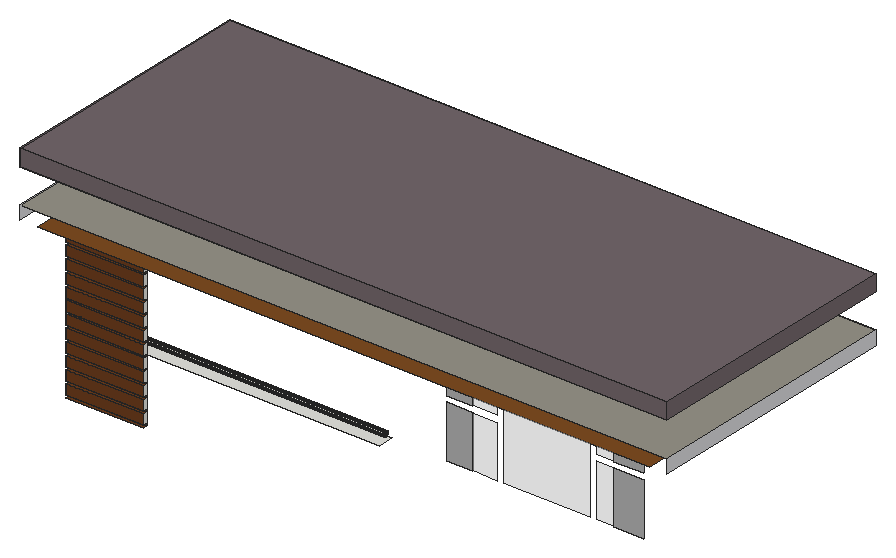
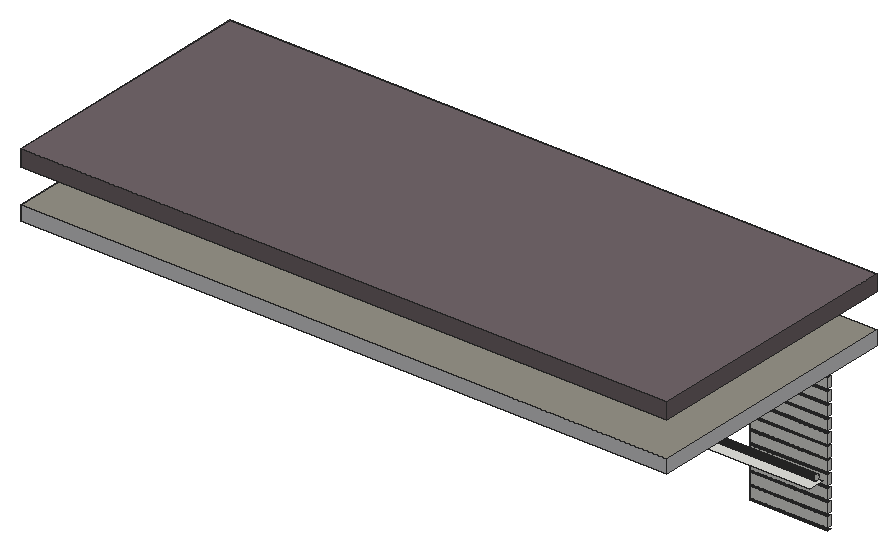
# SketchUp Ruby script. Lengths in inches.
U = 1.inch
M = Sketchup.active_model
def pt(a) = Geom::Point3d.new(a.map { |v| v * U })
def face(e, loops, mat)
  f = e.add_face(loops[0].map { |a| pt(a) })
  loops[1..].each { |l| e.add_face(l.map { |a| pt(a) }).erase! }
  f.material = f.back_material = mat if mat
  f
end
# faces: each face lists its corners as indices into pts; further lists are holes
def faces(e, pts, list, mat = nil) = list.each { |f| face(e, (f[0].is_a?(Array) ? f : [f]).map { |l| l.map { |i| pts[i] } }, mat) }
# xy, xz, yz: faces in a plane at the given z, y or x. An outline is a flat list of corners, or four numbers for a rectangle; further outlines are holes
def ring(l) = l.size == 4 ? [[l[0], l[1]], [l[2], l[1]], [l[2], l[3]], [l[0], l[3]]] : l.each_slice(2).to_a
def flat(e, list, mat, &to3) = list.each { |f| face(e, (f[0].is_a?(Array) ? f : [f]).map { |l| ring(l).map { |u, v| to3.(u, v) } }, mat) }
def xy(e, z, list, mat = nil) = flat(e, list, mat) { |x, y| [x, y, z] }
def xz(e, y, list, mat = nil) = flat(e, list, mat) { |x, z| [x, y, z] }
def yz(e, x, list, mat = nil) = flat(e, list, mat) { |y, z| [x, y, z] }
def lines(e, pts, list) = list.each { |a, b| e.add_line(pt(pts[a]), pt(pts[b])) }
# prism: a flat outline (further loops are holes) pulled along v
def prism(e, loops, v, mat = nil)
  f = face(e, loops, mat); d = Geom::Vector3d.new(v.map { |x| x * U })
  f.pushpull(f.normal.samedirection?(d) ? d.length : -d.length)
end
def box(e, o, s, mat = nil) = prism(e, [[o, [o[0] + s[0], o[1], o[2]], [o[0] + s[0], o[1] + s[1], o[2]], [o[0], o[1] + s[1], o[2]]]], [0, 0, s[2]], mat)
def at(x, y, z, deg = 0) = Geom::Transformation.translation(pt([x, y, z])) * Geom::Transformation.rotation(ORIGIN, Z_AXIS, deg.degrees)
def axes(o, x, y, z) = Geom::Transformation.new([*x, 0, *y, 0, *z, 0, *pt(o).to_a, 1])
def part(name) = M.definitions.add(name)
# library, detail: a bought-in or finely detailed component or shape, given as its bounding box
def library(name, o, s) = part(name).tap { |d| box(d.entities, o, s) }
def detail(e, o, s) = box(e.add_group.entities, o, s)
def put(e, d, t, mat = nil) = e.add_instance(d, t).tap { |i| i.material = mat if mat }
def group(e, t, mat = nil) = e.add_group.tap { |g| g.transformation = t; g.material = mat if mat }.entities
root = M.entities
M.materials.add("[Asphalt New]").color = [114, 102, 106]
M.materials.add("[Blinds Vertical Pattern]").color = [212, 212, 214]
M.materials.add("[Blinds Vertical Stripe Gray]1").color = [175, 175, 175]
M.materials.add("[Color M07]").color = [58, 58, 58]
M.materials.add("[Formica Graystone]3").color = [149, 146, 135]
M.materials.add("[Formica Laminate Dark]").color = [50, 53, 60]
M.materials.add("[Quartz Light Brown]").color = [224, 207, 171]
M.materials.add("[Terrazzo Tile Light]").color = [219, 217, 210]
M.materials.add("[Translucent Glass Gray]1").color = [224, 224, 224]
M.materials["[Translucent Glass Gray]1"].alpha = 0.5
M.materials.add("[Wood Cherry Original]").color = [107, 60, 29]
M.materials.add("[Wood Floor Parquet]").color = [124, 76, 33]
xy(root,275.9375,[[110.71,220.49,195.83,224.74]],"[Wood Cherry Original]")
xy(root,278.71,[[110.71,220.49,195.02,224.74],[195.02,220.49,195.83,224.74]],"[Wood Cherry Original]")
xy(root,289.6875,[[110.71,220.49,195.83,224.74]],"[Wood Cherry Original]")
xy(root,292.46,[[110.71,220.49,195.02,224.74],[195.02,220.49,195.83,224.74]],"[Wood Cherry Original]")
xy(root,303.4375,[[110.71,220.49,195.83,224.74]],"[Wood Cherry Original]")
xy(root,306.21,[[110.71,220.49,195.02,224.74],[195.02,220.49,195.83,224.74]],"[Wood Cherry Original]")
xy(root,317.1875,[[110.71,220.49,195.83,224.74]],"[Wood Cherry Original]")
xy(root,319.83,[[110.71,220.49,195.02,224.74],[195.02,220.49,195.83,224.74]],"[Wood Cherry Original]")
xy(root,330.8125,[[110.71,220.49,195.83,224.74]],"[Wood Cherry Original]")
xy(root,333.46,[[110.71,220.49,195.02,224.74],[195.02,220.49,195.83,224.74]],"[Wood Cherry Original]")
xy(root,334.75,[[102.3,241.34,438.59,258.82]])
xy(root,344.4375,[[110.71,220.49,195.83,224.74]],"[Wood Cherry Original]")
xy(root,347.08,[[110.71,220.49,195.02,224.74],[195.02,220.49,195.83,224.74]],"[Wood Cherry Original]")
xy(root,358.0625,[[110.71,220.49,195.83,224.74]],"[Wood Cherry Original]")
xy(root,360.71,[[110.71,220.49,195.02,224.74],[195.02,220.49,195.83,224.74]],"[Wood Cherry Original]")
xy(root,371.6875,[[110.71,220.49,195.83,224.74]],"[Wood Cherry Original]")
xy(root,374.33,[[110.71,220.49,195.02,224.74],[195.02,220.49,195.83,224.74]],"[Wood Cherry Original]")
xy(root,385.3125,[[110.71,220.49,195.83,224.74]],"[Wood Cherry Original]")
xy(root,387.96,[[110.71,220.49,195.02,224.74],[195.02,220.49,195.83,224.74]],"[Wood Cherry Original]")
xy(root,398.9375,[[110.71,220.49,195.83,224.74]],"[Wood Cherry Original]")
xy(root,401.58,[[110.71,220.49,195.02,224.74],[195.02,220.49,195.83,224.74]],"[Wood Cherry Original]")
xy(root,412.5625,[[110.71,220.49,195.83,224.74]],"[Wood Cherry Original]")
xy(root,415.21,[[110.71,220.49,195.02,224.74],[195.02,220.49,195.83,224.74]],"[Wood Cherry Original]")
xy(root,426.1875,[[110.71,220.49,195.83,224.74]],"[Wood Cherry Original]")
xy(root,428.83,[[110.71,220.49,195.02,224.74],[195.02,220.49,195.83,224.74]],"[Wood Cherry Original]")
xy(root,430,[[488.69,241.34,724.51,258.97]],"[Quartz Light Brown]")
xy(root,439.8125,[[110.71,220.49,195.83,224.74]],"[Wood Cherry Original]")
xy(root,442.46,[[110.71,220.49,195.02,224.74],[195.02,220.49,195.83,224.74]],"[Wood Cherry Original]")
xy(root,453.4375,[[83.3125,217.06,102.3,233.68],[102.3,217.06,102.3,233.68,204.43,233.68,204.43,217.06,195.83,217.06,195.83,224.74,110.71,224.74,110.71,217.06],[110.71,220.49,195.83,224.74],[110.71,220.49,195.83,224.74],[83.3125,233.68,102.3,241.34],
  [83.3125,241.34,102.3,355.28],[438.59,241.34,774.88,305.05],[774.88,241.34,793.87,305.05],[438.59,305.05,455.13,355.28],[455.13,305.05,774.88,355.28],
  [774.88,305.05,793.87,355.28],[83.3125,355.28,102.3,479.71],[102.3,355.28,438.59,460.72],[438.59,355.28,455.13,460.72],[455.13,355.28,774.88,460.72],
  [774.88,355.28,793.87,479.71],[102.3,460.72,438.59,479.71],[438.59,460.72,455.13,479.71],[455.13,460.72,774.88,479.71]])
xy(root,453.4375,[[102.3,191.84,102.3,217.06,110.71,217.06,110.71,220.49,195.83,220.49,195.83,217.06,204.43,217.06,204.43,233.68,102.3,233.68,102.3,355.28,438.59,355.28,438.59,241.34,774.88,241.34,774.88,191.84]],"[Wood Floor Parquet]")
xy(root,468.5,[[164.19,296.67,679.38,375.05]])
xy(root,468.5,[[[83.3125,191.84,793.87,479.71],[164.19,296.67,679.38,375.05]]],"[Formica Graystone]3")
xy(root,506.5,[[164.19,296.67,679.38,375.05]])
xy(root,506.5,[[83.3125,191.84,83.3125,479.71,164.19,479.71,164.19,296.67,679.38,296.67,679.38,479.71,793.87,479.71,793.87,191.84],[164.19,375.05,679.38,479.71]],"[Asphalt New]")
xy(root,524.25,[[83.3125,191.84,793.87,479.71]],"[Asphalt New]")
xz(root,191.84,[[83.3125,506.5,793.87,524.25]],"[Asphalt New]")
xz(root,220.49,[[110.71,278.71,195.83,289.6875],[110.71,292.46,195.83,303.4375],[110.71,306.21,195.83,317.1875],[110.71,319.83,195.83,330.8125],[110.71,333.46,195.83,344.4375],
  [110.71,347.08,195.83,358.0625],[110.71,360.71,195.83,371.6875],[110.71,374.33,195.83,385.3125],[110.71,387.96,195.83,398.9375],[110.71,401.58,195.83,412.5625],
  [110.71,415.21,195.83,426.1875],[110.71,428.83,195.83,439.8125],[110.71,442.46,195.83,453.4375]],"[Wood Cherry Original]")
xz(root,224.74,[[110.71,278.71,195.83,289.6875],[110.71,292.46,195.83,303.4375],[110.71,306.21,195.83,317.1875],[110.71,319.83,195.83,330.8125],[110.71,333.46,195.83,344.4375],
  [110.71,347.08,195.83,358.0625],[110.71,360.71,195.83,371.6875],[110.71,374.33,195.83,385.3125],[110.71,387.96,195.83,398.9375],[110.71,401.58,195.83,412.5625],
  [110.71,415.21,195.83,426.1875],[110.71,428.83,195.83,439.8125],[110.71,442.46,195.83,453.4375]])
xz(root,224.74,[[110.71,275.9375,195.83,278.71],[110.71,289.6875,195.83,292.46],[110.71,303.4375,195.83,306.21],[110.71,317.1875,195.83,319.83],[110.71,330.8125,195.83,333.46],
  [110.71,344.4375,195.83,347.08],[110.71,358.0625,195.83,360.71],[110.71,371.6875,195.83,374.33],[110.71,385.3125,195.83,387.96],[110.71,398.9375,195.83,401.58],
  [110.71,412.5625,195.83,415.21],[110.71,426.1875,195.83,428.83],[110.71,439.8125,195.83,442.46]],"[Color M07]")
xz(root,258.97,[[497.89,332.38,526.43,390.39],[682.12,332.38,715.3125,390.39],[497.89,396.84,526.43,420.81],[682.12,396.84,715.3125,420.81]],"[Blinds Vertical Stripe Gray]1")
xz(root,258.97,[[526.43,332.38,554.98,390.39],[561.48,332.38,656.23,420.81],[662.73,332.38,682.12,390.39],[526.43,396.84,554.98,420.81],[662.73,396.84,682.12,420.81]],"[Translucent Glass Gray]1")
xz(root,296.67,[[164.19,468.5,679.38,506.5]],"[Formica Laminate Dark]")
xz(root,375.05,[[164.19,468.5,679.38,506.5]],"[Formica Laminate Dark]")
xz(root,479.71,[[83.3125,506.5,793.87,524.25]],"[Asphalt New]")
xz(root,479.71,[[83.3125,453.4375,793.87,468.5]],"[Blinds Vertical Pattern]")
yz(root,83.3125,[[191.84,506.5,479.71,524.25]],"[Asphalt New]")
yz(root,83.3125,[[191.84,453.4375,479.71,468.5]],"[Blinds Vertical Pattern]")
yz(root,102.3,[[250.08,339.44,249.34,339.54,248.64,339.83,248.05,340.28,247.59,340.88,247.3,341.57,247.21,342.32,247.3,343.06,247.59,343.75,248.05,344.35,248.64,344.81,249.34,345.09,250.08,345.19,250.83,345.09,251.52,344.81,252.11,344.35,252.57,343.75,252.86,343.06,252.96,342.32,252.86,341.57,252.57,340.88,252.11,340.28,251.52,339.83,250.83,339.54]])
yz(root,110.71,[[220.49,278.71,224.74,289.6875],[220.49,292.46,224.74,303.4375],[220.49,306.21,224.74,317.1875],[220.49,319.83,224.74,330.8125],[220.49,333.46,224.74,344.4375],
  [220.49,347.08,224.74,358.0625],[220.49,360.71,224.74,371.6875],[220.49,374.33,224.74,385.3125],[220.49,387.96,224.74,398.9375],[220.49,401.58,224.74,412.5625],
  [220.49,415.21,224.74,426.1875],[220.49,428.83,224.74,439.8125],[220.49,442.46,224.74,453.4375]])
yz(root,164.19,[[296.67,468.5,375.05,506.5]],"[Formica Laminate Dark]")
yz(root,195.83,[[220.49,278.71,224.74,289.6875],[220.49,292.46,224.74,303.4375],[220.49,306.21,224.74,317.1875],[220.49,319.83,224.74,330.8125],[220.49,333.46,224.74,344.4375],
  [220.49,347.08,224.74,358.0625],[220.49,360.71,224.74,371.6875],[220.49,374.33,224.74,385.3125],[220.49,387.96,224.74,398.9375],[220.49,401.58,224.74,412.5625],
  [220.49,415.21,224.74,426.1875],[220.49,428.83,224.74,439.8125],[220.49,442.46,224.74,453.4375]])
yz(root,679.38,[[296.67,468.5,375.05,506.5]],"[Formica Laminate Dark]")
yz(root,793.87,[[191.84,506.5,479.71,524.25]],"[Asphalt New]")
yz(root,793.87,[[191.84,453.4375,479.71,468.5]],"[Blinds Vertical Pattern]")
p = [[102.3,249.34,339.54],[102.3,250.08,339.44],[438.59,250.08,339.44],[438.59,249.34,339.54],[102.3,250.83,339.54],[438.59,250.83,339.54],
  [102.3,248.64,339.83],[438.59,248.64,339.83],[102.3,251.52,339.83],[438.59,251.52,339.83],[102.3,248.05,340.28],[438.59,248.05,340.28],
  [102.3,252.11,340.28],[438.59,252.11,340.28],[102.3,247.59,340.88],[438.59,247.59,340.88],[102.3,252.57,340.88],[438.59,252.57,340.88],
  [102.3,247.3,341.57],[438.59,247.3,341.57],[102.3,252.86,341.57],[438.59,252.86,341.57],[102.3,247.21,342.32],[438.59,247.21,342.32],
  [102.3,252.96,342.32],[438.59,252.96,342.32],[102.3,247.3,343.06],[438.59,247.3,343.06],[102.3,252.86,343.06],[438.59,252.86,343.06],
  [102.3,247.59,343.75],[438.59,247.59,343.75],[102.3,252.57,343.75],[438.59,252.57,343.75],[102.3,248.05,344.35],[438.59,248.05,344.35],
  [102.3,252.11,344.35],[438.59,252.11,344.35],[102.3,248.64,344.81],[438.59,248.64,344.81],[102.3,251.52,344.81],[438.59,251.52,344.81],
  [102.3,249.34,345.09],[438.59,249.34,345.09],[102.3,250.83,345.09],[438.59,250.83,345.09],[102.3,250.08,345.19],[438.59,250.08,345.19]]
faces(root,p,[[0,1,2,3],[1,4,5,2],[6,0,3,7],[4,8,9,5],[10,6,7,11],[8,12,13,9],[14,10,11,15],[12,16,17,13],
  [18,14,15,19],[16,20,21,17],[22,18,19,23],[20,24,25,21],[26,22,23,27],[24,28,29,25],[30,26,27,31],[28,32,33,29],
  [34,30,31,35],[32,36,37,33],[38,34,35,39],[36,40,41,37],[42,38,39,43],[40,44,45,41],[46,42,43,47],[44,46,47,45]],"[Terrazzo Tile Light]")
